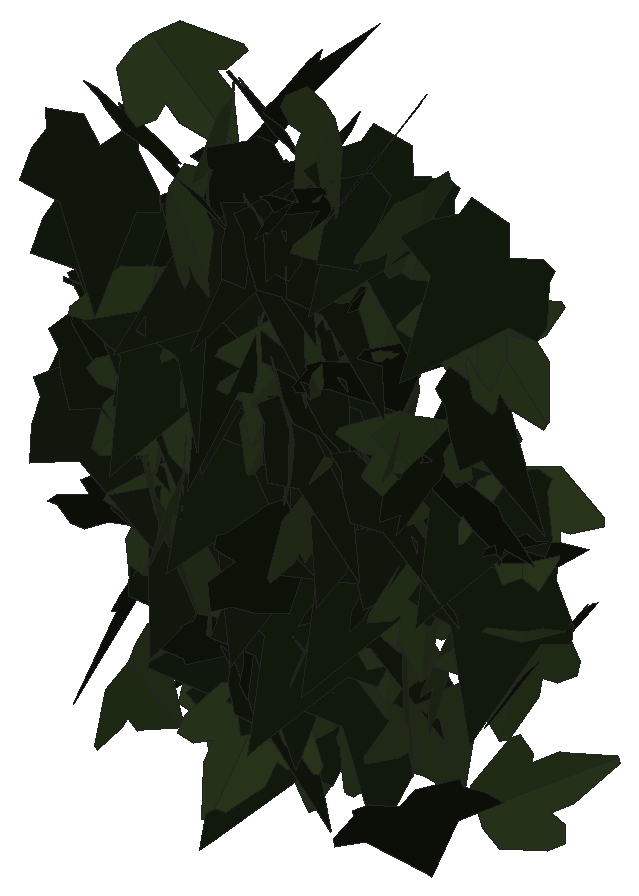
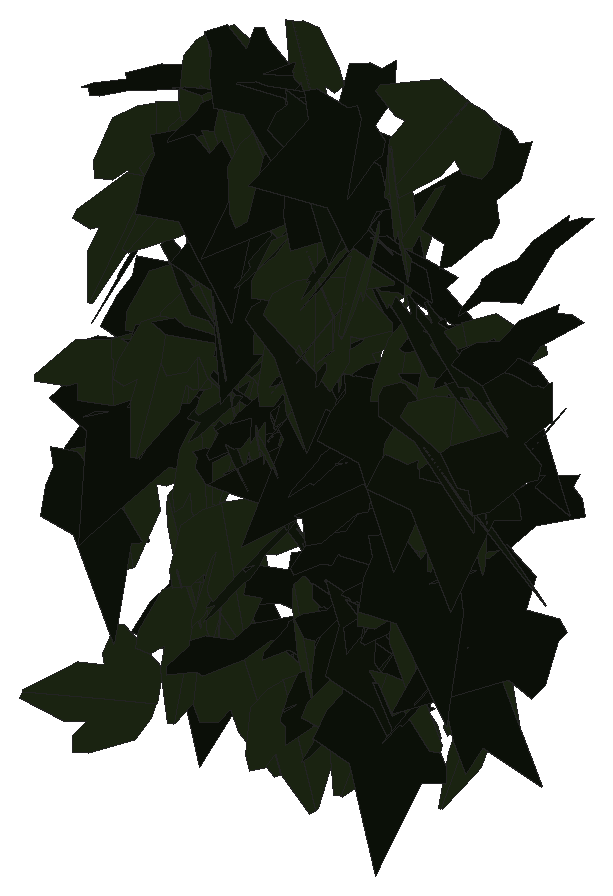
# SketchUp Ruby script. Lengths in inches.
U = 1.inch
M = Sketchup.active_model
def pt(a) = Geom::Point3d.new(a.map { |v| v * U })
def face(e, loops, mat)
  f = e.add_face(loops[0].map { |a| pt(a) })
  loops[1..].each { |l| e.add_face(l.map { |a| pt(a) }).erase! }
  f.material = f.back_material = mat if mat
  f
end
# faces: each face lists its corners as indices into pts; further lists are holes
def faces(e, pts, list, mat = nil) = list.each { |f| face(e, (f[0].is_a?(Array) ? f : [f]).map { |l| l.map { |i| pts[i] } }, mat) }
# xy, xz, yz: faces in a plane at the given z, y or x. An outline is a flat list of corners, or four numbers for a rectangle; further outlines are holes
def ring(l) = l.size == 4 ? [[l[0], l[1]], [l[2], l[1]], [l[2], l[3]], [l[0], l[3]]] : l.each_slice(2).to_a
def flat(e, list, mat, &to3) = list.each { |f| face(e, (f[0].is_a?(Array) ? f : [f]).map { |l| ring(l).map { |u, v| to3.(u, v) } }, mat) }
def xy(e, z, list, mat = nil) = flat(e, list, mat) { |x, y| [x, y, z] }
def xz(e, y, list, mat = nil) = flat(e, list, mat) { |x, z| [x, y, z] }
def yz(e, x, list, mat = nil) = flat(e, list, mat) { |y, z| [x, y, z] }
def lines(e, pts, list) = list.each { |a, b| e.add_line(pt(pts[a]), pt(pts[b])) }
# prism: a flat outline (further loops are holes) pulled along v
def prism(e, loops, v, mat = nil)
  f = face(e, loops, mat); d = Geom::Vector3d.new(v.map { |x| x * U })
  f.pushpull(f.normal.samedirection?(d) ? d.length : -d.length)
end
def box(e, o, s, mat = nil) = prism(e, [[o, [o[0] + s[0], o[1], o[2]], [o[0] + s[0], o[1] + s[1], o[2]], [o[0], o[1] + s[1], o[2]]]], [0, 0, s[2]], mat)
def at(x, y, z, deg = 0) = Geom::Transformation.translation(pt([x, y, z])) * Geom::Transformation.rotation(ORIGIN, Z_AXIS, deg.degrees)
def axes(o, x, y, z) = Geom::Transformation.new([*x, 0, *y, 0, *z, 0, *pt(o).to_a, 1])
def part(name) = M.definitions.add(name)
# library, detail: a bought-in or finely detailed component or shape, given as its bounding box
def library(name, o, s) = part(name).tap { |d| box(d.entities, o, s) }
def detail(e, o, s) = box(e.add_group.entities, o, s)
def put(e, d, t, mat = nil) = e.add_instance(d, t).tap { |i| i.material = mat if mat }
def group(e, t, mat = nil) = e.add_group.tap { |g| g.transformation = t; g.material = mat if mat }.entities
root = M.entities
M.materials.add("efeu1").color = [18, 25, 13]
M.materials.add("efeu2").color = [43, 57, 29]
c1 = part("ivyleaf_9")
p = [[1.54,2.16,1.25],[1.36,2.04,1.19],[-0.21,0.99,0.68],[-0.71,1.11,0.82],[-0.85,0.86,0.67],[-0.8,0.17,0.21],
  [-0.9,-0.01,0.1],[-0.67,-0.16,-0.02],[-0.08,-0.08,-0.05],[-0.03,-0.6,-0.4],[0.65,-0.88,-0.66],[0.83,-0.6,-0.49],
  [1.29,-0.42,-0.43],[1.8125,-0.07,-0.26],[1.21,0.44,0.15]]
faces(c1.entities,p,[[0,1,2,3,4,5,6,7,8,9,10,11,12,13,14]],"efeu1")
c2 = part("ivyleaf_10")
p = [[0,0.5,-0.03],[-0.0625,2.02,-0.43],[-0.19,2.01,-0.46],[-0.54,1.05,-0.29],[-0.52,0.625,-0.18],[-0.83,0.76,-0.28],
  [-1.16,0.64,-0.33],[-1.15,0.33,-0.24],[-0.77,-0.39,0.02],[-0.3,-0.51,0.16],[0.04,-0.48,0.23],[-0.02,2.01,-0.4375],
  [-0.06,2.01,-0.43],[0.04,-0.49,0.23],[0.67,-0.49,0.14],[1.38,0.36,-0.2],[1.375,0.51,-0.24],[0.81,0.65,-0.19],
  [0.62,0.59,-0.15],[0.6,1.09,-0.28],[0.5,1.23,-0.31]]
faces(c2.entities,p,[[0,1,2,3,4,5,6,7,8,9,10],[11,12,0,13,14,15,16,17,18,19,20]],"efeu2")
put(root,c1,axes([40.57,222.06,243.66],[0.41774,0.22902,0.15182],[0.11148,0.11124,-0.47455],[-0.25114,0.43032,0.04188]))
put(root,c1,axes([40.59,222.02,245.2],[0.26568,-0.40705,-0.11713],[-0.03559,0.11633,-0.48498],[0.42207,0.26604,0.03284]))
put(root,c1,axes([40.71,222.16,246.44],[-0.06068,-0.4911,-0.07169],[0.02532,0.06907,-0.49456],[0.49566,-0.06365,0.01648]))
put(root,c1,axes([40.47,222.22,245.51],[0.42978,-0.1592,0.19987],[0.23581,0.09648,-0.43021],[0.09841,0.46406,0.15801]))
put(root,c1,axes([40.92,222.38,243.02],[-0.27047,0.24039,-0.34505],[0.23268,-0.25619,-0.36087],[-0.35029,-0.35578,0.02671]))
put(root,c1,axes([40.73,221.89,247.15],[-0.00658,-0.49915,0.02835],[0.00658,-0.02844,-0.49915],[0.49991,-0.00619,0.00694]))
put(root,c1,axes([40.72,221.99,244.78],[-0.04875,-0.42008,-0.26675],[0.07847,0.25819,-0.42093],[0.49139,-0.08291,0.04076]))
put(root,c1,axes([41.21,222.28,244.96],[-0.4174,0.26946,0.05627],[-0.04592,0.03261,-0.49682],[-0.27142,-0.41991,-0.00247]))
put(root,c1,axes([41.11,222.36,245.11],[0.08551,0.49169,0.03048],[-0.13658,0.05338,-0.47801],[-0.47332,0.07343,0.14344]))
put(root,c1,axes([41.23,221.79,245.72],[0.0954,0.08783,-0.48289],[-0.40513,-0.26361,-0.12799],[-0.27707,0.41569,0.02086]))
put(root,c2,axes([41.09,222.41,245.55],[-0.42242,-0.26672,-0.02063],[0.01106,0.02111,-0.49943],[0.26729,-0.42239,-0.01194]))
put(root,c1,axes([41.29,222.58,244.12],[-0.07761,0.49091,-0.0546],[0.00566,-0.05438,-0.497],[-0.49391,-0.07776,0.00289]))
put(root,c1,axes([41.37,222.24,246.36],[-0.42348,0.26032,-0.05384],[0.04136,-0.03552,-0.49702],[-0.26259,-0.42541,0.00855]))
put(root,c2,axes([40.95,222.14,244.74],[0.2549,-0.35588,0.2416],[0.28651,-0.069,-0.40392],[0.32084,0.34436,0.16875]))
put(root,c1,axes([41.52,222.1875,245.42],[-0.12241,0.4353,0.21338],[-0.18699,0.16065,-0.435],[-0.44727,-0.1863,0.12346]))
put(root,c2,axes([41.35,222.28,243.87],[-0.16703,-0.41186,0.22906],[-0.03493,-0.23154,-0.44178],[0.46998,-0.16358,0.04858]))
put(root,c2,axes([41.3125,221.88,246.01],[-0.2486,-0.42328,0.09506],[0.02258,-0.12203,-0.48435],[0.43323,-0.23653,0.07979]))
put(root,c2,axes([41.29,221.69,242.34],[-0.0151,-0.40398,-0.29423],[0.09533,0.28663,-0.39844],[0.4906,-0.06813,0.06837]))
put(root,c1,axes([41.09,222.56,243.02],[0.15245,-0.47599,0.01394],[0.01102,-0.01111,-0.49976],[0.47606,0.15269,0.0071]))
put(root,c2,axes([41.38,222.51,243.9],[-0.30614,-0.3942,-0.0297],[0.02004,0.02204,-0.49911],[0.39481,-0.30679,0.00231]))
put(root,c2,axes([41.52,221.6875,245.15],[0.39947,0.01012,-0.30054],[-0.29515,0.10879,-0.38865],[0.05752,0.48792,0.09289]))
put(root,c1,axes([41.63,222.22,246.34],[-0.4007,0.29631,-0.04042],[0.03519,-0.0204,-0.49834],[-0.29698,-0.40222,-0.00451]))
put(root,c2,axes([41.3,222.03,245.28],[0.42754,-0.22768,0.12396],[0.12449,-0.0294,-0.48336],[0.2274,0.44418,0.03155]))
put(root,c1,axes([41.07,221.85,247.64],[0.33686,-0.32423,0.17719],[0.17735,-0.06846,-0.46245],[0.32414,0.37441,0.06888]))
put(root,c2,axes([41.47,222.19,245.02],[0.38311,-0.26362,-0.18367],[-0.03656,0.24821,-0.4325],[0.3192,0.34482,0.1709]))
put(root,c1,axes([41.6,222.63,242.43],[0.02694,0.49471,0.06739],[0.00243,0.06735,-0.49544],[-0.49927,0.02702,0.00122]))
put(root,c1,axes([41.33,222.2,245.12],[0.08973,-0.49187,-0.00321],[-0.01223,0.00103,-0.49985],[0.49173,0.08979,-0.01184]))
put(root,c1,axes([41.46,222.48,243.63],[-0.18659,-0.45218,0.10352],[0.00208,-0.11239,-0.4872],[0.46388,-0.18138,0.04382]))
put(root,c1,axes([41.68,222.41,245.44],[0.05191,0.49667,0.02497],[-0.05505,0.0307,-0.49601],[-0.49424,0.04875,0.05787]))
put(root,c1,axes([41.63,222.01,245.71],[-0.31479,-0.38735,0.02948],[-0.01966,-0.02201,-0.49913],[0.38797,-0.3154,-0.00137]))
put(root,c2,axes([41.79,221.65,244.39],[0.14367,-0.39544,-0.27016],[-0.07033,0.26157,-0.42028],[0.47372,0.15876,0.01954]))
put(root,c2,axes([41.49,221.87,248.33],[0.34832,0.19009,0.3042],[0.19411,0.25669,-0.38266],[-0.30165,0.38468,0.10502]))
put(root,c2,axes([41.81,221.65,243.89],[-0.45561,0.20523,-0.01749],[0.01625,-0.00652,-0.49969],[-0.20533,-0.45589,-0.00073]))
put(root,c2,axes([41.77,222.15,246],[-0.00593,-0.49101,-0.09419],[0.13312,0.08924,-0.47362],[0.48192,-0.03069,0.12967]))
put(root,c2,axes([41.82,222.57,242.55],[-0.41653,-0.24111,-0.13553],[0.15878,-0.00784,-0.47405],[0.22647,-0.43796,0.0831]))
put(root,c1,axes([41.99,222.41,242.81],[0.12495,0.13879,0.46382],[-0.02954,0.48031,-0.13577],[-0.48323,0.00653,0.12822]))
put(root,c2,axes([41.88,222.17,247.75],[0.19978,-0.45835,0.00106],[0.05426,0.0225,-0.49654],[0.45513,0.19851,0.05873]))
put(root,c2,axes([41.93,221.55,247.14],[-0.17119,0.44908,0.13792],[-0.04543,0.13028,-0.48059],[-0.46758,-0.17707,-0.0038]))
put(root,c1,axes([42.24,221.95,246.66],[-0.49409,-0.04503,0.06203],[-0.06223,-0.0006,-0.49611],[0.04476,-0.49797,-0.00501]))
put(root,c1,axes([41.89,222.21,245.87],[-0.10353,-0.48892,0.01547],[-0.00218,-0.01535,-0.49976],[0.48916,-0.10355,0.00105]))
put(root,c1,axes([42.21,221.95,242.85],[0.23487,0.31021,-0.31402],[-0.20184,-0.24086,-0.38891],[-0.39255,0.30945,0.01209]))
put(root,c1,axes([42.19,222.24,244.72],[-0.34306,-0.35708,0.06929],[0.02502,-0.11819,-0.48518],[0.36288,-0.32943,0.09897]))
put(root,c1,axes([42.28,222.11,242.5],[-0.00596,-0.11773,0.48591],[0.06963,0.48101,0.1174],[-0.49509,0.06906,0.01066]))
put(root,c2,axes([42.14,222.09,242.31],[0.49827,-0.03996,-0.0112],[-0.01029,0.01182,-0.49975],[0.0402,0.49826,0.01096]))
put(root,c1,axes([42.63,222.03,242.8125],[-0.39653,0.14286,0.26899],[-0.25706,0.07985,-0.42136],[-0.16335,-0.47246,0.01012]))
put(root,c1,axes([42.27,221.8,246.01],[-0.39749,0.03929,-0.30076],[0.30057,-0.01555,-0.39927],[-0.04073,-0.49821,-0.01125]))
put(root,c1,axes([42.3,222.3,247.88],[-0.15387,0.33872,-0.33406],[-0.13738,0.3045,0.37203],[0.45547,0.20627,-0.00064]))
put(root,c2,axes([42.29,222.12,246.93],[-0.36101,0.34565,0.01415],[-0.00828,0.0118,-0.49979],[-0.34584,-0.36109,-0.0028]))
put(root,c1,axes([42.57,222.09,247.58],[0.03957,0.29632,-0.40079],[-0.22819,-0.34667,-0.27884],[-0.44313,0.20498,0.1078]))
put(root,c1,axes([42.15,222.49,245.07],[0.05429,-0.49584,-0.03452],[0.00756,0.03554,-0.49868],[0.49699,0.05362,0.01136]))
put(root,c1,axes([42.3,222.35,244.02],[-0.17818,-0.46595,0.0338],[0.0082,-0.03929,-0.49839],[0.4671,-0.17705,0.02164]))
put(root,c1,axes([42.47,222.36,242.13],[-0.37737,-0.3275,0.01839],[-0.02158,-0.00319,-0.49952],[0.3273,-0.3778,-0.01172]))
put(root,c2,axes([42.43,221.92,242.2],[0.38583,0.26412,-0.17714],[-0.1563,-0.08506,-0.46726],[-0.27696,0.41594,0.01693]))
put(root,c1,axes([42.26,222.29,242.32],[0.23891,-0.43257,0.0762],[0.07045,-0.04788,-0.49269],[0.43354,0.24615,0.03807]))
put(root,c1,axes([42.24,222.125,248.1],[0.42319,-0.25748,0.0679],[0.06294,-0.02716,-0.49528],[0.25874,0.42774,0.00943]))
put(root,c1,axes([42.39,222.25,245.01],[0.48567,0.11881,-0.00307],[-0.00317,0.00002,-0.49999],[-0.11881,0.48568,0.00077]))
put(root,c1,axes([42.24,222.41,244.6875],[0.40914,-0.1579,0.24014],[0.25439,0.00454,-0.43042],[0.13375,0.47439,0.08406]))
put(root,c1,axes([42.5,222.4,243.15],[-0.05901,-0.49374,-0.05233],[0.01696,0.05066,-0.49714],[0.49622,-0.06044,0.01077]))
put(root,c1,axes([42.42,222.1,246.83],[0.18244,-0.46548,0.00674],[0.00054,-0.00703,-0.49995],[0.46553,0.18243,-0.00206]))
put(root,c2,axes([42.74,222.0625,245.62],[-0.13405,-0.44032,0.19532],[-0.02759,-0.19539,-0.45942],[0.4809,-0.13395,0.02808]))
put(root,c1,axes([42.91,222.34,245.69],[-0.06409,0.38042,0.31808],[-0.12447,0.29811,-0.38162],[-0.48,-0.1281,0.05649]))
put(root,c1,axes([42.78,221.9375,247.26],[-0.45412,0.03669,-0.20598],[0.18908,-0.13876,-0.44158],[-0.08957,-0.47896,0.11216]))
put(root,c1,axes([42.42,222.59,242.47],[0.42446,-0.17198,-0.20063],[0.19583,-0.05018,0.45731],[-0.17743,-0.4668,0.02476]))
put(root,c2,axes([42.81,222.01,245.95],[-0.18115,-0.42139,0.19903],[-0.03545,-0.20046,-0.45668],[0.46468,-0.17957,0.04275]))
put(root,c1,axes([42.94,221.86,247.54],[-0.04018,0.42463,0.26091],[-0.0996,0.24963,-0.42162],[-0.48833,-0.08586,0.06453]))
put(root,c2,axes([42.76,222.43,243.0625],[0.1963,-0.45612,-0.05849],[-0.00663,0.06078,-0.49625],[0.45981,0.1956,0.01781]))
put(root,c2,axes([42.82,222.53,242.1],[-0.18369,-0.456,0.09123],[-0.01213,-0.09336,-0.49106],[0.46488,-0.18262,0.02323]))
put(root,c2,axes([42.8,222.22,246.09],[-0.31666,-0.38694,-0.00103],[0.04181,-0.03289,-0.49716],[0.38468,-0.31495,0.05318]))
put(root,c1,axes([42.56,222.01,246.91],[0.30277,-0.3973,-0.02207],[-0.00433,0.02445,-0.49938],[0.39789,0.30259,0.01136]))
put(root,c2,axes([42.86,222.13,246.55],[-0.38748,-0.31568,0.01441],[0.05246,-0.08673,-0.48962],[0.31163,-0.37792,0.10033]))
put(root,c2,axes([42.9,222.28,245.66],[-0.1364,-0.48097,0.00813],[0.00334,-0.00939,-0.4999],[0.48102,-0.13631,0.00577]))
put(root,c1,axes([42.64,222.35,245.93],[0.18734,-0.46197,0.03854],[0.02081,-0.03314,-0.49847],[0.46311,0.18837,0.00681]))
put(root,c1,axes([43.01,222.27,243.32],[-0.38714,-0.31627,-0.00979],[0.0018,0.01327,-0.49982],[0.31642,-0.38704,-0.00914]))
put(root,c1,axes([42.73,221.36,244.08],[0.10912,0.30062,-0.38435],[0.03809,0.38739,0.31381],[0.48646,-0.09776,0.06164]))
put(root,c2,axes([43.21,221.36,245.51],[0.1013,-0.07772,-0.48342],[-0.21283,0.43759,-0.11495],[0.44095,0.22907,0.05557]))
put(root,c1,axes([42.88,222.28,245.38],[0.0862,-0.45564,-0.18698],[0.01098,0.19155,-0.46172],[0.49239,0.07549,0.04303]))
put(root,c2,axes([42.86,222.03,246.03],[-0.04489,-0.04586,-0.49587],[0.2833,-0.41181,0.01244],[-0.40954,-0.27984,0.06295]))
put(root,c1,axes([42.83,222.08,245.52],[0.33049,-0.37096,0.05626],[0.06475,-0.01745,-0.49548],[0.36957,0.33479,0.03651]))
put(root,c1,axes([42.95,221.92,245.23],[0.22996,-0.44023,-0.05761],[-0.02293,0.05302,-0.49665],[0.44339,0.23106,0.00419]))
put(root,c2,axes([43.43,222.47,242.28],[-0.42734,-0.10611,0.23691],[-0.22234,-0.08587,-0.43953],[0.13397,-0.48101,0.0262]))
put(root,c2,axes([43.2,221.7,244.64],[0.00325,-0.42914,-0.25657],[0.0802,0.2537,-0.42333],[0.49352,-0.0384,0.07048]))
put(root,c2,axes([43.33,221.69,248.33],[0.39082,-0.22073,-0.22031],[-0.13992,0.19157,-0.44014],[0.27872,0.40568,0.08797]))
put(root,c1,axes([43.06,221.82,247.47],[0.4802,0.13369,0.03915],[0.02869,0.04259,-0.49736],[-0.13632,0.47991,0.03324]))
put(root,c1,axes([43.27,222.39,244.89],[-0.17155,-0.46527,0.06396],[-0.00386,-0.0667,-0.49552],[0.46963,-0.17051,0.0193]))
put(root,c2,axes([43.23,222.39,244.54],[0.35828,-0.30465,0.16978],[0.15255,-0.082,-0.46905],[0.31363,0.3879,0.03419]))
put(root,c1,axes([43.12,222.12,246.75],[0.17774,-0.46042,0.08017],[0.08265,-0.05346,-0.49022],[0.45998,0.18751,0.0571]))
put(root,c2,axes([43.49,222.08,247.32],[-0.09657,-0.46667,0.15131],[0.00093,-0.15439,-0.47557],[0.49058,-0.09157,0.03069]))
put(root,c1,axes([43.37,222.64,242.64],[-0.19663,-0.44731,-0.10607],[0.07158,0.08417,-0.48764],[0.4541,-0.20696,0.03094]))
put(root,c1,axes([43.76,222.06,244.24],[-0.39167,0.31072,-0.00709],[0.00425,-0.00606,-0.49995],[-0.31077,-0.39169,0.00211]))
put(root,c1,axes([43.22,222.46,243.48],[0.26382,-0.4241,-0.02315],[0.03916,0.05142,-0.49581],[0.42292,0.2598,0.06034]))
put(root,c1,axes([43.79,221.93,248.2],[-0.22507,0.44404,-0.04658],[0.02324,-0.04043,-0.49782],[-0.44587,-0.22626,-0.00244]))
put(root,c1,axes([43.93,221.95,244.6],[-0.44972,0.16246,0.14614],[-0.14051,0.04111,-0.47809],[-0.16735,-0.47108,0.00868]))
put(root,c2,axes([43.68,222.4,243.55],[-0.30766,-0.38455,0.0864],[-0.00678,-0.10442,-0.48893],[0.39408,-0.30202,0.05904]))
put(root,c1,axes([43.66,221.76,246.16],[0.28049,0.41286,-0.02952],[-0.07184,0.01343,-0.49463],[-0.40764,0.28171,0.06686]))
put(root,c1,axes([43.7,222.125,244.21],[-0.38255,-0.32164,-0.01424],[0.01203,0.00782,-0.49979],[0.32173,-0.38274,0.00176]))
put(root,c2,axes([43.7,222.15,244.74],[-0.45178,0.21423,-0.00169],[0.00152,-0.00075,-0.5],[-0.21423,-0.45178,0.00003]))
put(root,c2,axes([43.88,222.19,245.57],[0.23421,-0.43895,-0.04963],[0.00262,0.05755,-0.49667],[0.44174,0.23239,0.02926]))
put(root,c2,axes([43.89,222.23,243.12],[-0.19911,0.4548,-0.05926],[-0.04859,-0.08516,-0.49029],[-0.45606,-0.18949,0.07811]))
put(root,c1,axes([43.94,222.11,247.87],[-0.39977,-0.29895,0.02856],[0.06611,-0.13398,-0.47716],[0.29294,-0.37773,0.14665]))
put(root,c1,axes([44.05,222.16,247.13],[0.00406,0.48265,-0.13051],[-0.0034,-0.13049,-0.48266],[-0.49997,0.00481,0.00222]))
put(root,c2,axes([43.875,222.0625,247.57],[0.49473,-0.07235,-0.00187],[-0.00198,-0.00063,-0.5],[0.07235,0.49474,-0.00091]))
put(root,c2,axes([44.18,222.01,245.46],[-0.32676,-0.31375,0.21163],[-0.14797,-0.15144,-0.45296],[0.34833,-0.35865,0.00612]))
put(root,c2,axes([44.04,222.37,242.59],[-0.24277,-0.41601,-0.13417],[0.06236,0.11894,-0.48163],[0.43264,-0.25058,-0.00587]))
put(root,c1,axes([43.74,222,244.93],[0.25422,-0.42838,0.04314],[0.09115,0.00459,-0.4916],[0.42079,0.25781,0.08042]))
put(root,c2,axes([44.22,221.86,247.26],[-0.31519,-0.35052,0.1667],[-0.09131,-0.14176,-0.47071],[0.37725,-0.32717,0.02535]))
put(root,c1,axes([43.92,221.95,247.71],[-0.00466,-0.48111,-0.13606],[0.01184,0.13592,-0.48103],[0.49984,-0.00771,0.01013]))
put(root,c2,axes([44.15,222.1,244.14],[-0.00508,-0.49751,0.04961],[0.11315,-0.04947,-0.48451],[0.487,0.0063,0.11309]))
put(root,c2,axes([44.24,222.36,243.4375],[0.21013,-0.4536,0.00978],[0.00859,-0.0068,-0.49988],[0.45362,0.21025,0.00494]))
put(root,c2,axes([44.3,221.8,247.89],[-0.03488,-0.49759,-0.03451],[0.00007,0.03458,-0.4988],[0.49878,-0.0348,-0.00234]))
put(root,c1,axes([44.36,221.51,242.15],[0.20924,0.44891,-0.06857],[-0.04662,-0.05386,-0.4949],[-0.45172,0.21349,0.01932]))
put(root,c2,axes([44.38,222,245.59],[-0.42737,-0.25939,0.00829],[-0.00895,-0.00124,-0.49992],[0.25937,-0.42745,-0.00359]))
put(root,c2,axes([44.19,222.05,246.96],[-0.19618,-0.2916,-0.35565],[0.25675,0.25135,-0.34771],[0.38157,-0.31905,0.05111]))
put(root,c2,axes([44.38,222.36,245.1875],[-0.14577,-0.42977,-0.20987],[0.081,0.19405,-0.45363],[0.47137,-0.16625,0.01305]))
put(root,c1,axes([44.63,221.68,245.64],[-0.3572,0.34956,-0.01479],[0.00884,-0.01211,-0.49978],[-0.34976,-0.3573,0.00247]))
put(root,c1,axes([44.72,222.39,245.13],[-0.3708,-0.33535,-0.00681],[0.0073,0.00208,-0.49994],[0.33534,-0.37086,0.00335]))
put(root,c2,axes([44.51,222.77,241.7],[-0.04329,-0.14321,0.47709],[0.1566,0.4507,0.14949],[-0.47287,0.16236,0.00583]))
put(root,c1,axes([44.77,221.78,245.29],[0.39253,0.11417,-0.28789],[-0.28616,-0.04408,-0.40764],[-0.11846,0.48479,0.03074]))
put(root,c1,axes([44.76,222.12,244.4],[0.28949,0.40588,0.03817],[0.01856,0.03364,-0.49852],[-0.40725,0.29005,0.00441]))
put(root,c2,axes([44.84,221.95,247.06],[-0.33709,-0.36908,0.0123],[0.04328,-0.05603,-0.49496],[0.36674,-0.33263,0.06972]))
put(root,c2,axes([44.8,222.29,246.52],[0.02203,0.4409,0.23477],[-0.02112,0.23561,-0.4405],[-0.49907,0.00949,0.029]))
put(root,c1,axes([45.16,222.41,243.49],[-0.12018,0.48164,0.05984],[-0.00051,0.06152,-0.4962],[-0.48534,-0.11932,-0.0143]))
put(root,c1,axes([44.8125,221.91,246.26],[0.29334,-0.35004,-0.20351],[-0.13673,0.15091,-0.45665],[0.38112,0.32356,-0.00718]))
put(root,c1,axes([44.93,222.25,244.27],[-0.19968,-0.45731,-0.03147],[0.01455,0.02798,-0.499],[0.45816,-0.2002,0.00214]))
put(root,c2,axes([44.91,222.48,244.97],[0.33752,0.36874,-0.01075],[-0.00094,-0.01372,-0.49981],[-0.36889,0.33741,-0.00857]))
put(root,c2,axes([45.125,222.17,243.69],[-0.3173,-0.37947,0.07296],[-0.04808,-0.0549,-0.49465],[0.38342,-0.32092,-0.00165]))
put(root,c1,axes([45.07,222.01,247.55],[-0.35715,-0.32902,0.11913],[0.0172,-0.18653,-0.46358],[0.3495,-0.32704,0.14456]))
